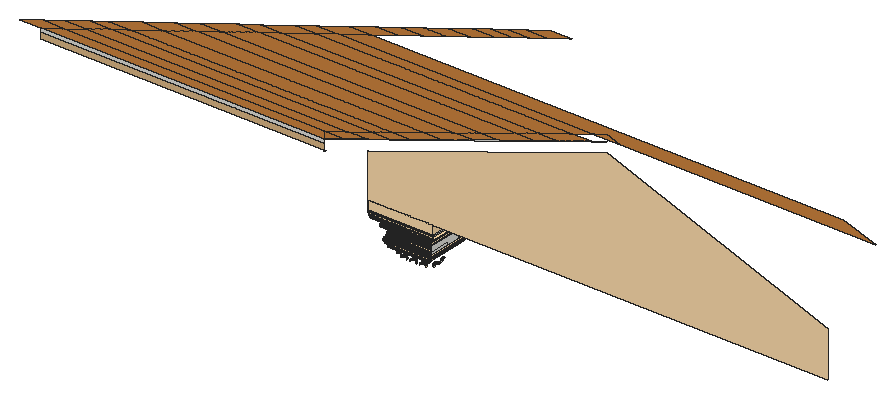
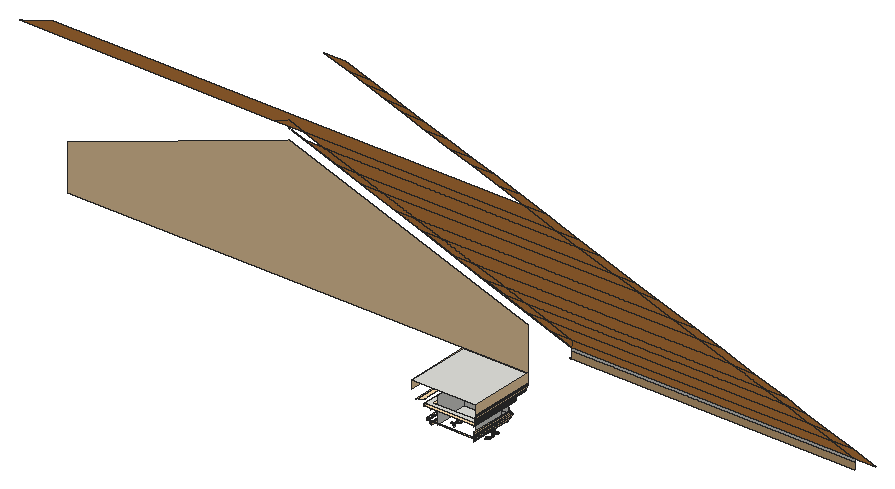
# SketchUp Ruby script. Lengths in inches.
U = 1.inch
M = Sketchup.active_model
def pt(a) = Geom::Point3d.new(a.map { |v| v * U })
def face(e, loops, mat)
  f = e.add_face(loops[0].map { |a| pt(a) })
  loops[1..].each { |l| e.add_face(l.map { |a| pt(a) }).erase! }
  f.material = f.back_material = mat if mat
  f
end
# faces: each face lists its corners as indices into pts; further lists are holes
def faces(e, pts, list, mat = nil) = list.each { |f| face(e, (f[0].is_a?(Array) ? f : [f]).map { |l| l.map { |i| pts[i] } }, mat) }
# xy, xz, yz: faces in a plane at the given z, y or x. An outline is a flat list of corners, or four numbers for a rectangle; further outlines are holes
def ring(l) = l.size == 4 ? [[l[0], l[1]], [l[2], l[1]], [l[2], l[3]], [l[0], l[3]]] : l.each_slice(2).to_a
def flat(e, list, mat, &to3) = list.each { |f| face(e, (f[0].is_a?(Array) ? f : [f]).map { |l| ring(l).map { |u, v| to3.(u, v) } }, mat) }
def xy(e, z, list, mat = nil) = flat(e, list, mat) { |x, y| [x, y, z] }
def xz(e, y, list, mat = nil) = flat(e, list, mat) { |x, z| [x, y, z] }
def yz(e, x, list, mat = nil) = flat(e, list, mat) { |y, z| [x, y, z] }
def lines(e, pts, list) = list.each { |a, b| e.add_line(pt(pts[a]), pt(pts[b])) }
# prism: a flat outline (further loops are holes) pulled along v
def prism(e, loops, v, mat = nil)
  f = face(e, loops, mat); d = Geom::Vector3d.new(v.map { |x| x * U })
  f.pushpull(f.normal.samedirection?(d) ? d.length : -d.length)
end
def box(e, o, s, mat = nil) = prism(e, [[o, [o[0] + s[0], o[1], o[2]], [o[0] + s[0], o[1] + s[1], o[2]], [o[0], o[1] + s[1], o[2]]]], [0, 0, s[2]], mat)
def at(x, y, z, deg = 0) = Geom::Transformation.translation(pt([x, y, z])) * Geom::Transformation.rotation(ORIGIN, Z_AXIS, deg.degrees)
def axes(o, x, y, z) = Geom::Transformation.new([*x, 0, *y, 0, *z, 0, *pt(o).to_a, 1])
def part(name) = M.definitions.add(name)
# library, detail: a bought-in or finely detailed component or shape, given as its bounding box
def library(name, o, s) = part(name).tap { |d| box(d.entities, o, s) }
def detail(e, o, s) = box(e.add_group.entities, o, s)
def put(e, d, t, mat = nil) = e.add_instance(d, t).tap { |i| i.material = mat if mat }
def group(e, t, mat = nil) = e.add_group.tap { |g| g.transformation = t; g.material = mat if mat }.entities
root = M.entities
M.materials.add("[0033_NavajoWhite]").color = [255, 222, 173]
M.materials.add("[0036_BurlyWood]").color = [222, 184, 135]
M.materials.add("[0040_Peru]").color = [205, 133, 63]
xy(root,95.99,[[110.21,8.1,123.2,14.59]])
xy(root,96.66,[[[109.62,7.51,123.79,21.68],[109.69,7.58,123.72,21.61]]],"[0033_NavajoWhite]")
xy(root,100.56,[[[109.03,6.92,124.38,22.27],[110.21,8.1,123.2,21.09]]],"[0033_NavajoWhite]")
xy(root,101.46,[[[109.03,6.92,124.38,22.27],[110.21,8.1,123.2,21.09]]])
xy(root,102.72,[[108.83,6.72,109.03,6.92,124.38,6.92,124.58,6.72]])
xy(root,102.72,[[108.04,5.93,108.04,23.25,108.83,22.47,109.03,22.27,109.03,6.92],[108.04,5.93,108.83,6.72,124.58,6.72,125.37,5.93],[125.37,5.93,124.38,6.92,124.38,22.27,124.58,22.47,125.37,23.25]],"[0033_NavajoWhite]")
xy(root,102.86,[[111,9.67,122.41,14.59]])
xy(root,105.42,[[108.83,6.72,124.58,14.59]])
xy(root,108.125,[[106.86,4.75,126.55,24.44]])
xz(root,4.75,[[93.16,116.81,93.71,117,93.16,117],[6.32,119,93.16,120],[93.16,119.98,93.21,120,93.16,120],[93.16,120,93.21,120,120.1,129.23,120.04,129.23,113.85,127.11,106.79,124.68,99.27,122.1],[120.04,129.23,120.1,129.23,139.33,135.83,139.26,135.83,129.4375,132.46],
  [139.26,135.83,139.33,135.83,147.21,138.54,147.13,138.54],[147.13,138.54,147.21,138.54,164.92,144.62,164.84,144.62,157.86,142.22],[164.84,144.62,164.92,144.62,180,149.8,179.96,149.82,175.27,148.21]])
xz(root,4.75,[[106.86,105.42,126.55,108.125],[106.86,108.125,247.8,108.125,247.8,122.125,179.96,146.625,106.86,121.52]],"[0033_NavajoWhite]")
xz(root,4.75,[[6.32,117,93.16,119]],"[0036_BurlyWood]")
xz(root,4.75,[[0,120,6.32,120,13.35,122.34,7.02,122.34],[6.32,120,93.16,120,93.16,122.1,13.35,122.34],[93.16,120,99.27,122.1,93.16,122.1],[93.16,122.1,100.6875,124.68,20.37,124.68,13.35,122.34],[93.16,122.1,99.27,122.1,106.79,124.68,100.6875,124.68],
  [7.02,122.34,13.35,122.34,20.37,124.68,14.04,124.68],[14.04,124.68,20.37,124.68,27.65,127.11,21.32,127.11],[20.37,124.68,100.6875,124.68,107.75,127.11,27.65,127.11],[100.6875,124.68,106.79,124.68,113.85,127.11,107.75,127.11],[21.32,127.11,27.65,127.11,33.71,129.13,27.39,129.13],
  [27.65,127.11,107.75,127.11,113.9375,129.23,33.71,129.13],[107.75,127.11,113.85,127.11,120.04,129.23,113.9375,129.23],[27.39,129.13,33.71,129.13,43.71,132.46,37.38,132.46],[33.71,129.13,113.9375,129.23,123.33,132.46,43.71,132.46],[113.9375,129.23,120.04,129.23,129.4375,132.46,123.33,132.46],
  [37.38,132.46,43.71,132.46,53.83,135.83,47.5,135.83],[43.71,132.46,123.33,132.46,133.15,135.83,53.83,135.83],[123.33,132.46,129.4375,132.46,139.26,135.83,133.15,135.83],[47.5,135.83,53.83,135.83,61.94,138.54,55.62,138.54],[53.83,135.83,133.15,135.83,141.03,138.54,61.94,138.54],
  [133.15,135.83,139.26,135.83,147.13,138.54,141.03,138.54],[55.62,138.54,61.94,138.54,73,142.22,66.67,142.22],[61.94,138.54,141.03,138.54,151.75,142.22,73,142.22],[141.03,138.54,147.13,138.54,157.86,142.22,151.75,142.22],[66.67,142.22,73,142.22,80.19,144.62,73.87,144.62],
  [73,142.22,151.75,142.22,158.73,144.62,80.19,144.62],[151.75,142.22,157.86,142.22,164.84,144.62,158.73,144.62],[73.87,144.62,80.19,144.62,90.94,148.21,84.62,148.21],[80.19,144.62,158.73,144.62,169.17,148.21,90.94,148.21],[158.73,144.62,164.84,144.62,175.27,148.21,169.17,148.21],
  [84.62,148.21,90.94,148.21,97.46,150.38,91.14,150.38],[90.94,148.21,169.17,148.21,175.49,150.38,97.46,150.38],[91.14,150.38,97.46,150.38,107.66,153.78,101.33,153.78],[97.46,150.38,175.49,150.38,180,151.93,184.29,150.38,262.54,150.38,252.34,153.78,107.66,153.78],[175.49,150.38,184.29,150.38,180,151.93],
  [101.33,153.78,107.66,153.78,115.67,156.45,109.34,156.45],[109.34,156.45,115.67,156.45,123.61,159.09,117.28,159.09],[117.28,159.09,123.61,159.09,130.36,161.35,124.04,161.35],[124.04,161.35,130.36,161.35,137.99,163.89,131.67,163.89],[131.67,163.89,137.99,163.89,145.25,166.31,138.93,166.31],
  [138.93,166.31,145.25,166.31,150.49,168.05,144.16,168.05],[144.16,168.05,150.49,168.05,156.26,169.98,149.93,169.98],[149.93,169.98,156.26,169.98,161.41,171.69,155.08,171.69],[155.08,171.69,161.41,171.69,169.18,174.29,162.86,174.29]],"[0040_Peru]")
xz(root,6.72,[[108.83,102.72,124.58,105.42]])
xz(root,7.11,[[109.22,101.95,124.19,101.95,124.1875,102.09,109.23,102.09],[109.23,102.09,124.1875,102.09,124.19,102.23,109.22,102.23]],"[0033_NavajoWhite]")
xz(root,7.58,[[109.69,95.99,123.72,96.66]],"[0033_NavajoWhite]")
xz(root,8.1,[[110.21,94.95,123.2,95.1],[110.21,95.1,123.2,95.99],[110.21,95.99,123.2,97.5625],[110.21,97.5625,123.2,99.87],[110.21,99.87,123.2,100.56],
  [110.21,100.56,123.2,101.46]])
xz(root,9.67,[[111,94.95,122.41,102.86]])
yz(root,106.86,[[4.75,105.42,24.44,108.125]],"[0033_NavajoWhite]")
yz(root,110.21,[[8.1,95.99,14.59,97.5625]])
yz(root,111,[[9.67,94.95,19.51,102.86]])
yz(root,122.41,[[9.67,94.95,19.51,102.86]])
yz(root,123.2,[[8.1,95.99,14.59,97.5625]])
yz(root,126.55,[[4.75,105.42,24.44,108.125]],"[0033_NavajoWhite]")
p = [[112.83,9.92,92.48],[112.8,9.67,92.48],[112.77,9.67,92.25],[112.8,9.93,92.25],[114.7,9.93,92.25],[114.74,9.67,92.25],
  [114.7,9.67,92.48],[114.67,9.92,92.48],[115.79,9.92,92.48],[115.76,9.67,92.48],[115.72,9.67,92.25],[115.76,9.93,92.25],
  [117.66,9.93,92.25],[117.69,9.67,92.25],[117.66,9.67,92.48],[117.625,9.92,92.48],[118.74,9.92,92.48],[118.71,9.67,92.48],
  [118.67,9.67,92.25],[118.71,9.93,92.25],[120.61,9.93,92.25],[120.64,9.67,92.25],[120.61,9.67,92.48],[120.58,9.92,92.48],
  [112.9,10.16,92.25],[112.93,10.15,92.48],[114.58,10.15,92.48],[114.61,10.16,92.25],[115.85,10.16,92.25],[115.88,10.15,92.48],
  [117.53,10.15,92.48],[117.56,10.16,92.25],[118.81,10.16,92.25],[118.84,10.15,92.48],[120.48,10.15,92.48],[120.51,10.16,92.25],
  [113.06,10.37,92.25],[113.08,10.34,92.48],[114.43,10.34,92.48],[114.45,10.37,92.25],[116.01,10.37,92.25],[116.03,10.34,92.48],
  [117.38,10.34,92.48],[117.4,10.37,92.25],[118.96,10.37,92.25],[118.99,10.34,92.48],[120.33,10.34,92.48],[120.35,10.37,92.25],
  [113.26,10.52,92.25],[113.28,10.49,92.48],[114.23,10.49,92.48],[114.25,10.52,92.25],[116.21,10.52,92.25],[116.23,10.49,92.48],
  [117.18,10.49,92.48],[117.2,10.52,92.25],[119.17,10.52,92.25],[119.18,10.49,92.48],[120.13,10.49,92.48],[120.15,10.52,92.25],
  [113.5,10.62,92.25],[113.51,10.59,92.48],[114,10.59,92.48],[114.01,10.62,92.25],[116.45,10.62,92.25],[116.46,10.59,92.48],
  [116.95,10.59,92.48],[116.96,10.62,92.25],[119.4,10.62,92.25],[119.41,10.59,92.48],[119.9,10.59,92.48],[119.91,10.62,92.25],
  [113.75,10.66,92.25],[113.75,10.62,92.48],[116.71,10.66,92.25],[116.71,10.62,92.48],[119.66,10.66,92.25],[119.66,10.62,92.48],
  [112.93,9.89,92.7],[112.9,9.67,92.7],[114.61,9.67,92.7],[114.58,9.89,92.7],[115.88,9.89,92.7],[115.85,9.67,92.7],
  [117.56,9.67,92.7],[117.53,9.89,92.7],[118.84,9.89,92.7],[118.81,9.67,92.7],[120.51,9.67,92.7],[120.48,9.89,92.7],
  [113.01,10.1,92.7],[114.49,10.1,92.7],[115.97,10.1,92.7],[117.44,10.1,92.7],[118.92,10.1,92.7],[120.4,10.1,92.7],
  [113.15,10.27,92.7],[114.36,10.27,92.7],[116.1,10.27,92.7],[117.31,10.27,92.7],[119.06,10.27,92.7],[120.26,10.27,92.7],
  [113.33,10.41,92.7],[114.18,10.41,92.7],[116.28,10.41,92.7],[117.13,10.41,92.7],[119.23,10.41,92.7],[120.08,10.41,92.7],
  [113.53,10.49,92.7],[113.97,10.49,92.7],[116.49,10.49,92.7],[116.93,10.49,92.7],[119.4375,10.49,92.7],[119.88,10.49,92.7],
  [113.75,10.52,92.7],[116.71,10.52,92.7],[119.66,10.52,92.7],[111.25,10.6875,92.51],[111,10.66,92.51],[111,10.6875,92.74],
  [111.24,10.72,92.74],[111.47,10.82,92.74],[111.49,10.79,92.51],[121.92,10.79,92.51],[121.9375,10.82,92.74],[122.17,10.72,92.74],
  [122.16,10.6875,92.51],[122.41,10.66,92.51],[122.41,10.6875,92.74],[111.67,10.97,92.74],[111.69,10.94,92.51],[121.72,10.94,92.51],
  [121.74,10.97,92.74],[111.82,11.16,92.74],[111.85,11.15,92.51],[121.5625,11.15,92.51],[121.59,11.16,92.74],[111.92,11.39,92.74],
  [111.95,11.39,92.51],[121.46,11.39,92.51],[121.5,11.39,92.74],[111.95,11.64,92.74],[111.98,11.64,92.51],[121.43,11.64,92.51],
  [121.46,11.64,92.74],[111.92,11.89,92.74],[111.95,11.89,92.51],[121.46,11.89,92.51],[121.5,11.89,92.74],[111.82,12.12,92.74],
  [111.85,12.13,92.51],[121.5625,12.13,92.51],[121.59,12.12,92.74],[111.67,12.3125,92.74],[111.69,12.34,92.51],[121.72,12.34,92.51],
  [121.74,12.3125,92.74],[111.47,12.46,92.74],[111.49,12.49,92.51],[121.92,12.49,92.51],[121.9375,12.46,92.74],[111.24,12.56,92.74],
  [111.25,12.59,92.51],[122.16,12.59,92.51],[122.17,12.56,92.74],[111,12.59,92.74],[111,12.625,92.51],[122.41,12.59,92.74],
  [122.41,12.625,92.51],[111.25,13.64,92.51],[111,13.61,92.51],[111,13.64,92.74],[111.24,13.67,92.74],[111.47,13.77,92.74],
  [111.49,13.74,92.51],[121.92,13.74,92.51],[121.9375,13.77,92.74],[122.17,13.67,92.74],[122.16,13.64,92.51],[122.41,13.61,92.51],
  [122.41,13.64,92.74],[111.67,13.92,92.74],[111.69,13.9,92.51],[121.72,13.9,92.51],[121.74,13.92,92.74],[111.82,14.12,92.74],
  [111.85,14.1,92.51],[121.5625,14.1,92.51],[121.59,14.12,92.74],[111.92,14.35,92.74],[111.95,14.34,92.51],[121.46,14.34,92.51],
  [121.5,14.35,92.74],[111.95,14.59,92.74],[111.98,14.59,92.51],[121.43,14.59,92.51],[121.46,14.59,92.74],[113.08,9.85,92.89],
  [113.06,9.67,92.89],[114.45,9.67,92.89],[114.43,9.85,92.89],[116.03,9.85,92.89],[116.01,9.67,92.89],[117.4,9.67,92.89],
  [117.38,9.85,92.89],[118.99,9.85,92.89],[118.96,9.67,92.89],[120.35,9.67,92.89],[120.33,9.85,92.89],[113.15,10.02,92.89],
  [114.36,10.02,92.89],[116.1,10.02,92.89],[117.31,10.02,92.89],[119.06,10.02,92.89],[120.26,10.02,92.89],[113.26,10.16,92.89],
  [114.25,10.16,92.89],[116.21,10.16,92.89],[117.2,10.16,92.89],[119.17,10.16,92.89],[120.15,10.16,92.89],[113.41,10.27,92.89],
  [114.1,10.27,92.89],[116.36,10.27,92.89],[117.05,10.27,92.89],[119.3125,10.27,92.89],[120.01,10.27,92.89],[113.57,10.34,92.89],
  [113.75,10.37,92.89],[113.93,10.34,92.89],[116.53,10.34,92.89],[116.71,10.37,92.89],[116.89,10.34,92.89],[119.48,10.34,92.89],
  [119.66,10.37,92.89],[119.84,10.34,92.89],[111,10.79,92.96],[111.22,10.82,92.96],[111.42,10.9,92.96],[121.99,10.9,92.96],
  [122.19,10.82,92.96],[122.41,10.79,92.96],[111.6,11.04,92.96],[121.8125,11.04,92.96],[111.74,11.21,92.96],[121.68,11.21,92.96],
  [111.82,11.42,92.96],[121.59,11.42,92.96],[111.85,11.64,92.96],[121.5625,11.64,92.96],[111.82,11.86,92.96],[121.59,11.86,92.96],
  [111.74,12.07,92.96],[121.68,12.07,92.96],[111.6,12.24,92.96],[121.8125,12.24,92.96],[111.42,12.38,92.96],[121.99,12.38,92.96],
  [111.22,12.46,92.96],[122.19,12.46,92.96],[111,12.49,92.96],[122.41,12.49,92.96],[111,13.74,92.96],[111.22,13.77,92.96],
  [122.19,13.77,92.96],[122.41,13.74,92.96],[111.42,13.85,92.96],[121.99,13.85,92.96],[111.6,13.99,92.96],[121.8125,13.99,92.96],
  [111.74,14.17,92.96],[121.68,14.17,92.96],[111.82,14.37,92.96],[121.59,14.37,92.96],[111.85,14.59,92.96],[121.5625,14.59,92.96],
  [113.28,9.8,93.03],[113.26,9.67,93.03],[114.25,9.67,93.03],[114.23,9.8,93.03],[116.23,9.8,93.03],[116.21,9.67,93.03],
  [117.2,9.67,93.03],[117.18,9.8,93.03],[119.18,9.8,93.03],[119.17,9.67,93.03],[120.15,9.67,93.03],[120.13,9.8,93.03],
  [113.33,9.92,93.03],[114.18,9.92,93.03],[116.28,9.92,93.03],[117.13,9.92,93.03],[119.23,9.92,93.03],[120.08,9.92,93.03],
  [113.41,10.02,93.03],[114.1,10.02,93.03],[116.36,10.02,93.03],[117.05,10.02,93.03],[119.3125,10.02,93.03],[120.01,10.02,93.03],
  [113.51,10.1,93.03],[114,10.1,93.03],[116.46,10.1,93.03],[116.95,10.1,93.03],[119.41,10.1,93.03],[119.9,10.1,93.03],
  [113.625,10.15,93.03],[113.75,10.16,93.03],[113.88,10.15,93.03],[116.58,10.15,93.03],[116.71,10.16,93.03],[116.83,10.15,93.03],
  [119.53,10.15,93.03],[119.66,10.16,93.03],[119.79,10.15,93.03],[113.51,9.74,93.12],[113.5,9.67,93.12],[113.53,9.8,93.12],
  [114.01,9.67,93.12],[114,9.74,93.12],[113.97,9.8,93.12],[116.46,9.74,93.12],[116.45,9.67,93.12],[116.49,9.8,93.12],
  [116.93,9.8,93.12],[116.95,9.74,93.12],[116.96,9.67,93.12],[119.41,9.74,93.12],[119.4,9.67,93.12],[119.4375,9.8,93.12],
  [119.91,9.67,93.12],[119.9,9.74,93.12],[119.88,9.8,93.12],[113.57,9.85,93.12],[113.93,9.85,93.12],[116.53,9.85,93.12],
  [116.89,9.85,93.12],[119.48,9.85,93.12],[119.84,9.85,93.12],[113.625,9.89,93.12],[113.6875,9.92,93.12],[113.75,9.93,93.12],
  [113.82,9.92,93.12],[113.88,9.89,93.12],[116.58,9.89,93.12],[116.64,9.92,93.12],[116.71,9.93,93.12],[116.77,9.92,93.12],
  [116.83,9.89,93.12],[119.53,9.89,93.12],[119.59,9.92,93.12],[119.66,9.93,93.12],[119.72,9.92,93.12],[119.79,9.89,93.12],
  [111,10.94,93.15],[111.18,10.97,93.15],[111.35,11.04,93.15],[122.07,11.04,93.15],[122.23,10.97,93.15],[122.41,10.94,93.15],
  [111.49,11.15,93.15],[121.92,11.15,93.15],[111.6,11.29,93.15],[121.8125,11.29,93.15],[111.67,11.46,93.15],[121.74,11.46,93.15],
  [111.69,11.64,93.15],[121.72,11.64,93.15],[111.67,11.82,93.15],[121.74,11.82,93.15],[111.6,11.99,93.15],[121.8125,11.99,93.15],
  [111.49,12.13,93.15],[121.92,12.13,93.15],[111.35,12.24,93.15],[122.07,12.24,93.15],[111.18,12.3125,93.15],[122.23,12.3125,93.15],
  [111,12.34,93.15],[122.41,12.34,93.15],[111,13.9,93.15],[111.18,13.92,93.15],[122.23,13.92,93.15],[122.41,13.9,93.15],
  [111.35,13.99,93.15],[122.07,13.99,93.15],[111.49,14.1,93.15],[121.92,14.1,93.15],[111.6,14.24,93.15],[121.8125,14.24,93.15],
  [111.67,14.41,93.15],[121.74,14.41,93.15],[111.69,14.59,93.15],[121.72,14.59,93.15],[113.75,9.67,93.15],[116.71,9.67,93.15],
  [119.66,9.67,93.15],[111,11.15,93.29],[111.125,11.16,93.29],[122.29,11.16,93.29],[122.41,11.15,93.29],[111.24,11.21,93.29],
  [111.35,11.29,93.29],[122.07,11.29,93.29],[122.17,11.21,93.29],[111.42,11.39,93.29],[121.99,11.39,93.29],[111.47,11.51,93.29],
  [121.9375,11.51,93.29],[111.49,11.64,93.29],[121.92,11.64,93.29],[111.47,11.77,93.29],[121.9375,11.77,93.29],[111.42,11.89,93.29],
  [121.99,11.89,93.29],[111.35,11.99,93.29],[122.07,11.99,93.29],[111.24,12.07,93.29],[122.17,12.07,93.29],[111.125,12.12,93.29],
  [111,12.13,93.29],[122.29,12.12,93.29],[122.41,12.13,93.29],[111,14.1,93.29],[111.125,14.12,93.29],[111.24,14.17,93.29],
  [122.17,14.17,93.29],[122.29,14.12,93.29],[122.41,14.1,93.29],[111.35,14.24,93.29],[122.07,14.24,93.29],[111.42,14.35,93.29],
  [121.99,14.35,93.29],[111.47,14.47,93.29],[121.9375,14.47,93.29],[111.49,14.59,93.29],[121.92,14.59,93.29],[111,11.39,93.38],
  [111.0625,11.39,93.38],[122.35,11.39,93.38],[122.41,11.39,93.38],[111.125,11.42,93.38],[111.18,11.46,93.38],[122.23,11.46,93.38],
  [122.29,11.42,93.38],[111.22,11.51,93.38],[122.19,11.51,93.38],[111.24,11.57,93.38],[122.17,11.57,93.38],[111.25,11.64,93.38],
  [122.16,11.64,93.38],[111.24,11.71,93.38],[122.17,11.71,93.38],[111.22,11.77,93.38],[122.19,11.77,93.38],[111.125,11.86,93.38],
  [111.18,11.82,93.38],[122.23,11.82,93.38],[122.29,11.86,93.38],[111.0625,11.89,93.38],[111,11.89,93.38],[122.35,11.89,93.38],
  [122.41,11.89,93.38],[111,14.34,93.38],[111.0625,14.35,93.38],[111.125,14.37,93.38],[122.29,14.37,93.38],[122.35,14.35,93.38],
  [122.41,14.34,93.38],[111.18,14.41,93.38],[111.22,14.47,93.38],[122.19,14.47,93.38],[122.23,14.41,93.38],[111.24,14.53,93.38],
  [122.17,14.53,93.38],[111.25,14.59,93.38],[122.16,14.59,93.38],[111,11.64,93.41],[122.41,11.64,93.41],[111,14.59,93.41],
  [122.41,14.59,93.41],[110.2,8.09,95.25],[110.21,8.1,95.1],[123.2,8.1,95.1],[123.21,8.09,95.25],[110.18,8.06,95.4],
  [123.23,8.06,95.4],[110.15,8.03,95.53],[123.26,8.03,95.53],[110.15,21.15,95.53],[110.18,21.12,95.4],[123.23,21.12,95.4],
  [123.26,21.15,95.53],[110.11,8,95.66],[123.3,8,95.66],[110.11,21.1875,95.66],[123.3,21.1875,95.66],[110.0625,7.95,95.77],
  [123.35,7.95,95.77],[110.0625,21.24,95.77],[123.35,21.24,95.77],[110.01,7.9,95.86],[123.4,7.9,95.86],[109.89,7.78,95.98],
  [109.95,7.84,95.93],[123.46,7.84,95.93],[123.52,7.78,95.98],[109.89,21.41,95.98],[109.95,21.35,95.93],[123.46,21.35,95.93],
  [123.52,21.41,95.98],[109.86,7.74,95.99],[123.55,7.74,95.99],[109.48,7.37,96.79],[109.52,7.41,96.72],[123.89,7.41,96.72],
  [123.93,7.37,96.79],[109.57,7.45,96.68],[123.84,7.45,96.68],[109.48,21.82,96.79],[109.52,21.78,96.72],[109.57,21.73,96.68],
  [123.89,21.78,96.72],[123.93,21.82,96.79],[109.62,7.51,96.66],[123.79,7.51,96.66],[109.62,21.68,96.66],[109.45,7.34,96.89],
  [123.96,7.34,96.89],[109.45,21.85,96.89],[123.96,21.85,96.89],[109.43,7.32,96.99],[123.98,7.32,96.99],[109.43,21.87,96.99],
  [109.42,7.31,97.11],[123.99,7.31,97.11],[109.42,21.875,97.11],[109.43,7.32,97.23],[123.98,7.32,97.23],[109.43,21.87,97.23],
  [109.45,7.34,97.34],[123.96,7.34,97.34],[109.45,21.85,97.34],[109.48,7.37,97.43],[123.93,7.37,97.43],[109.48,21.82,97.43],
  [123.96,21.85,97.34],[123.93,21.82,97.43],[109.52,7.41,97.5],[123.89,7.41,97.5],[109.52,21.78,97.5],[123.89,21.78,97.5],
  [109.57,7.45,97.55],[123.84,7.45,97.55],[109.57,21.73,97.55],[109.62,7.51,97.5625],[123.79,7.51,97.5625],[109.62,21.68,97.5625],
  [109.72,7.61,97.74],[123.69,7.61,97.74],[109.72,21.58,97.74],[109.8125,7.7,97.93],[123.6,7.7,97.93],[109.9,7.78,98.14],
  [123.52,7.78,98.14],[109.9,21.4,98.14],[109.8125,21.49,97.93],[109.97,7.86,98.375],[123.44,7.86,98.375],[110.04,7.92,98.62],
  [123.375,7.92,98.62],[110.09,7.98,98.875],[123.32,7.98,98.875],[110.14,8.03,99.14],[123.27,8.03,99.14],[110.18,8.0625,99.42],
  [123.24,8.0625,99.42],[110.2,8.09,99.7],[123.21,8.09,99.7],[110.2,21.1,99.7],[110.18,21.12,99.42],[123.24,21.12,99.42],
  [123.21,21.1,99.7],[110.21,8.1,99.87],[123.2,8.1,99.87],[108.89,6.78,100.6875],[108.93,6.82,100.62],[124.48,6.82,100.62],
  [124.52,6.78,100.6875],[108.98,6.86,100.57],[124.43,6.86,100.57],[109.03,6.92,100.56],[124.38,6.92,100.56],[108.98,22.32,100.57],
  [109.03,22.27,100.56],[108.86,6.74,100.78],[124.55,6.74,100.78],[108.86,22.44,100.78],[108.89,22.41,100.6875],[108.84,6.73,100.89],
  [124.57,6.73,100.89],[108.84,22.46,100.89],[124.55,22.44,100.78],[124.57,22.46,100.89],[108.83,6.72,101.01],[124.58,6.72,101.01],
  [108.83,22.47,101.01],[108.84,6.73,101.125],[124.57,6.73,101.125],[108.84,22.46,101.125],[108.86,6.74,101.23],[124.55,6.74,101.23],
  [108.86,22.44,101.23],[124.57,22.46,101.125],[124.55,22.44,101.23],[108.89,6.78,101.33],[124.52,6.78,101.33],[108.89,22.41,101.33],
  [108.93,6.82,101.4],[124.48,6.82,101.4],[108.98,6.86,101.44],[124.43,6.86,101.44],[109.03,6.92,101.46],[124.38,6.92,101.46],
  [109.03,22.27,101.46],[108.98,22.32,101.44],[124.33,6.97,101.52],[109.08,6.97,101.52],[109.08,22.22,101.52],[124.33,22.22,101.52],
  [124.38,22.27,101.46],[124.28,7.02,101.6],[109.13,7.02,101.6],[109.13,22.17,101.6],[124.24,7.06,101.7],[109.17,7.06,101.7],
  [109.17,22.13,101.7],[124.21,7.09,101.82],[109.2,7.09,101.82],[109.2,22.1,101.82],[124.19,7.11,101.95],[109.22,7.11,101.95],
  [124.19,7.11,102.23],[124.21,7.09,102.36],[109.2,7.09,102.36],[109.22,7.11,102.23],[124.24,7.06,102.48],[109.17,7.06,102.48],
  [109.2,22.1,102.36],[109.17,22.13,102.48],[124.28,7.02,102.58],[109.13,7.02,102.58],[109.13,22.17,102.58],[124.33,6.97,102.66],
  [109.08,6.97,102.66],[109.08,22.22,102.66],[125.6875,5.61,102.73],[125.85,5.45,102.82],[107.57,5.45,102.82],[107.72,5.61,102.73],
  [107.57,23.73,102.82],[107.72,23.58,102.73],[125.6875,23.58,102.73],[125.85,23.73,102.82],[125.53,5.77,102.7],[107.88,5.77,102.7],
  [107.88,23.41,102.7],[125.37,5.93,102.72],[108.04,5.93,102.72],[108.04,23.25,102.72],[124.38,6.92,102.72],[109.03,6.92,102.72],
  [109.03,22.27,102.72],[124.38,22.27,102.72],[124.33,22.22,102.66],[125.99,5.3,102.96],[107.42,5.3,102.96],[107.42,23.88,102.96],
  [126.13,5.17,103.15],[107.28,5.17,103.15],[126.25,5.05,103.39],[107.16,5.05,103.39],[107.16,24.14,103.39],[107.28,24.02,103.15],
  [126.36,4.94,103.68],[107.05,4.94,103.68],[107.05,24.24,103.68],[126.44,4.86,103.99],[106.97,4.86,103.99],[126.51,4.79,104.33],
  [106.91,4.79,104.33],[106.91,24.39,104.33],[106.97,24.33,103.99],[126.54,4.75,104.6875],[106.87,4.75,104.6875],[106.87,24.43,104.6875],
  [126.56,4.74,105.05],[106.85,4.74,105.05],[126.55,4.75,105.42],[106.86,4.75,105.42],[106.86,24.44,105.42],[106.85,24.45,105.05]]
faces(root,p,[[0,1,2,3],[4,5,6,7],[8,9,10,11],[12,13,14,15],[16,17,18,19],[20,21,22,23],[0,3,24,25],[26,27,4,7],
  [8,11,28,29],[30,31,12,15],[16,19,32,33],[34,35,20,23],[25,24,36,37],[38,39,27,26],[29,28,40,41],[42,43,31,30],
  [33,32,44,45],[46,47,35,34],[37,36,48,49],[50,51,39,38],[41,40,52,53],[54,55,43,42],[45,44,56,57],[58,59,47,46],
  [49,48,60,61],[62,63,51,50],[53,52,64,65],[66,67,55,54],[57,56,68,69],[70,71,59,58],[61,60,72,73],[73,72,63,62],
  [65,64,74,75],[75,74,67,66],[69,68,76,77],[77,76,71,70],[78,79,1,0],[7,6,80,81],[82,83,9,8],[15,14,84,85],
  [86,87,17,16],[23,22,88,89],[78,0,25,90],[91,26,7,81],[82,8,29,92],[93,30,15,85],[86,16,33,94],[95,34,23,89],
  [90,25,37,96],[97,38,26,91],[92,29,41,98],[99,42,30,93],[94,33,45,100],[101,46,34,95],[96,37,49,102],[103,50,38,97],
  [98,41,53,104],[105,54,42,99],[100,45,57,106],[107,58,46,101],[102,49,61,108],[109,62,50,103],[104,53,65,110],[111,66,54,105],
  [106,57,69,112],[113,70,58,107],[108,61,73,114],[114,73,62,109],[110,65,75,115],[115,75,66,111],[112,69,77,116],[116,77,70,113],
  [197,198,79,78],[81,80,199,200],[201,202,83,82],[85,84,203,204],[205,206,87,86],[89,88,207,208],[197,78,90,209],[210,91,81,200],
  [201,82,92,211],[212,93,85,204],[205,86,94,213],[214,95,89,208],[209,90,96,215],[216,97,91,210],[211,92,98,217],[218,99,93,212],
  [213,94,100,219],[220,101,95,214],[215,96,102,221],[222,103,97,216],[217,98,104,223],[224,105,99,218],[219,100,106,225],[226,107,101,220],
  [221,102,108,227],[227,108,114,228],[228,114,109,229],[229,109,103,222],[223,104,110,230],[230,110,115,231],[231,115,111,232],[232,111,105,224],
  [225,106,112,233],[233,112,116,234],[234,116,113,235],[235,113,107,226],[276,277,198,197],[200,199,278,279],[280,281,202,201],[204,203,282,283],
  [284,285,206,205],[208,207,286,287],[276,197,209,288],[289,210,200,279],[280,201,211,290],[291,212,204,283],[284,205,213,292],[293,214,208,287],
  [288,209,215,294],[295,216,210,289],[290,211,217,296],[297,218,212,291],[292,213,219,298],[299,220,214,293],[294,215,221,300],[301,222,216,295],
  [296,217,223,302],[303,224,218,297],[298,219,225,304],[305,226,220,299],[300,221,227,306],[306,227,228,307],[307,228,229,308],[308,229,222,301],
  [302,223,230,309],[309,230,231,310],[310,231,232,311],[311,232,224,303],[304,225,233,312],[312,233,234,313],[313,234,235,314],[314,235,226,305],
  [315,316,277,276],[315,276,288,317],[279,278,318,319],[320,289,279,319],[321,322,281,280],[321,280,290,323],[324,291,283,325],[283,282,326,325],
  [327,328,285,284],[327,284,292,329],[287,286,330,331],[332,293,287,331],[317,288,294,333],[334,295,289,320],[323,290,296,335],[336,297,291,324],
  [329,292,298,337],[338,299,293,332],[333,294,300,339],[339,300,306,340],[340,306,307,341],[342,308,301,343],[341,307,308,342],[343,301,295,334],
  [335,296,302,344],[344,302,309,345],[345,309,310,346],[346,310,311,347],[348,303,297,336],[347,311,303,348],[337,298,304,349],[349,304,312,350],
  [350,312,313,351],[352,314,305,353],[351,313,314,352],[353,305,299,338],[315,394,316],[394,315,317],[394,317,333],[394,333,339],
  [394,339,340],[394,340,341],[319,318,394],[394,320,319],[394,334,320],[394,343,334],[394,342,343],[394,341,342],
  [321,395,322],[395,321,323],[395,323,335],[395,335,344],[395,344,345],[395,345,346],[325,326,395],[395,324,325],
  [395,336,324],[395,348,336],[395,347,348],[395,346,347],[327,396,328],[396,327,329],[396,329,337],[396,337,349],
  [396,349,350],[396,350,351],[331,330,396],[396,332,331],[396,338,332],[396,353,338],[396,352,353],[396,351,352],
  [481,482,483,484],[485,481,484,486],[487,485,486,488],[487,489,490,485],[486,491,492,488],[493,487,488,494],[493,495,489,487],[488,492,496,494],
  [497,493,494,498],[497,499,495,493],[494,496,500,498],[501,497,498,502],[503,504,505,506],[503,507,508,504],[504,501,502,505],[505,509,510,506],
  [511,503,506,512],[513,514,515,516],[514,517,518,515],[513,519,520,514],[514,520,521,517],[515,522,523,516],[517,524,525,518],[517,521,526,524],
  [527,513,516,528],[527,529,519,513],[516,523,530,528],[531,527,528,532],[531,533,529,527],[534,531,532,535],[534,536,533,531],[537,534,535,538],
  [537,539,536,534],[540,537,538,541],[540,542,539,537],[543,540,541,544],[543,545,542,540],[541,546,547,544],[548,543,544,549],[548,550,545,543],
  [544,547,551,549],[552,548,549,553],[552,554,550,548],[555,552,553,556],[555,557,554,552],[558,555,556,559],[558,560,557,555],[561,558,559,562],
  [563,561,562,564],[563,565,566,561],[567,563,564,568],[569,567,568,570],[571,569,570,572],[573,571,572,574],[575,573,574,576],[577,575,576,578],
  [579,580,575,577],[576,581,582,578],[583,577,578,584],[585,586,587,588],[586,589,590,587],[589,591,592,590],[589,593,594,591],[595,585,588,596],
  [595,597,598,585],[599,595,596,600],[599,601,597,595],[596,602,603,600],[604,599,600,605],[604,606,601,599],[607,604,605,608],[607,609,606,604],
  [610,607,608,611],[610,612,609,607],[613,614,611,608],[615,610,611,616],[615,617,612,610],[618,615,616,619],[620,618,619,621],[622,620,621,623],
  [622,624,625,620],[623,626,627,622],[626,631,632,627],[631,634,635,632],[634,637,638,635],[637,640,641,638],[642,643,644,645],[643,646,647,644],
  [646,650,651,647],[650,653,654,651],[656,657,658,659],[658,660,661,659],[656,662,663,657],[664,656,659,665],[659,661,666,665],[667,664,665,668],
  [665,666,669,668],[653,670,671,654],[657,675,676,658],[676,677,660,658],[675,678,679,676],[678,680,681,679],[681,682,683,679],[680,684,685,681],
  [685,686,682,681],[684,687,688,685],[687,689,690,688],[690,691,692,688],[689,693,694,690],[694,695,691,690],[693,696,697,694],[696,698,699,697],
  [699,700,701,697]],"[0033_NavajoWhite]")
faces(root,p,[[117,118,119,120],[121,122,117,120],[123,124,125,126],[127,126,125,128],[129,130,122,121],[131,132,124,123],[133,134,130,129],[135,136,132,131],
  [137,138,134,133],[139,140,136,135],[141,142,138,137],[143,144,140,139],[145,146,142,141],[147,148,144,143],[149,150,146,145],[151,152,148,147],
  [153,154,150,149],[155,156,152,151],[157,158,154,153],[159,160,156,155],[161,162,158,157],[163,164,160,159],[161,165,166,162],[167,164,163,168],
  [169,170,171,172],[173,174,169,172],[175,176,177,178],[179,178,177,180],[181,182,174,173],[183,184,176,175],[185,186,182,181],[187,188,184,183],
  [189,190,186,185],[191,192,188,187],[193,194,190,189],[195,196,192,191],[120,119,236,237],[238,121,120,237],[124,239,240,125],[128,125,240,241],
  [242,129,121,238],[132,243,239,124],[244,133,129,242],[136,245,243,132],[246,137,133,244],[140,247,245,136],[248,141,137,246],[144,249,247,140],
  [250,145,141,248],[148,251,249,144],[252,149,145,250],[152,253,251,148],[254,153,149,252],[156,255,253,152],[256,157,153,254],[160,257,255,156],
  [258,161,157,256],[164,259,257,160],[258,260,165,161],[261,259,164,167],[172,171,262,263],[180,177,264,265],[266,173,172,263],[176,267,264,177],
  [268,181,173,266],[184,269,267,176],[270,185,181,268],[188,271,269,184],[272,189,185,270],[192,273,271,188],[274,193,189,272],[196,275,273,192],
  [237,236,354,355],[356,238,237,355],[239,357,358,240],[241,240,358,359],[360,242,238,356],[243,361,357,239],[362,244,242,360],[245,363,361,243],
  [364,246,244,362],[247,365,363,245],[366,248,246,364],[249,367,365,247],[368,250,248,366],[251,369,367,249],[370,252,250,368],[253,371,369,251],
  [372,254,252,370],[255,373,371,253],[374,256,254,372],[257,375,373,255],[376,258,256,374],[259,377,375,257],[376,378,260,258],[379,377,259,261],
  [263,262,380,381],[265,264,382,383],[384,266,263,381],[267,385,382,264],[386,268,266,384],[269,387,385,267],[388,270,268,386],[271,389,387,269],
  [390,272,270,388],[273,391,389,271],[392,274,272,390],[275,393,391,273],[355,354,397,398],[359,358,399,400],[401,356,355,398],[402,360,356,401],
  [361,403,404,357],[357,404,399,358],[405,362,360,402],[363,406,403,361],[407,364,362,405],[365,408,406,363],[409,366,364,407],[367,410,408,365],
  [411,368,366,409],[369,412,410,367],[413,370,368,411],[371,414,412,369],[415,372,370,413],[373,416,414,371],[417,374,372,415],[375,418,416,373],
  [419,420,378,376],[419,376,374,417],[377,421,418,375],[422,421,377,379],[381,380,423,424],[425,384,381,424],[385,426,427,382],[383,382,427,428],
  [429,386,384,425],[387,430,426,385],[431,388,386,429],[389,432,430,387],[433,390,388,431],[391,434,432,389],[435,392,390,433],[393,436,434,391],
  [398,397,437,438],[400,399,439,440],[441,401,398,438],[442,402,401,441],[403,443,444,404],[404,444,439,399],[445,405,402,442],[406,446,443,403],
  [447,407,405,445],[408,448,446,406],[449,409,407,447],[410,450,448,408],[451,411,409,449],[412,452,450,410],[453,413,411,451],[414,454,452,412],
  [455,417,415,456],[456,415,413,453],[416,457,454,414],[418,458,457,416],[459,460,420,419],[459,419,417,455],[421,461,458,418],[462,461,421,422],
  [424,423,463,464],[465,425,424,464],[426,466,467,427],[428,427,467,468],[469,429,425,465],[470,431,429,469],[432,471,472,430],[430,472,466,426],
  [473,433,431,470],[434,474,471,432],[475,435,433,473],[436,476,474,434],[438,437,477],[477,441,438],[477,442,441],[443,478,444],
  [440,439,478],[444,478,439],[477,445,442],[477,447,445],[446,478,443],[448,478,446],[477,449,447],[477,451,449],
  [477,453,451],[477,456,453],[477,455,456],[477,459,455],[459,477,460],[450,478,448],[452,478,450],[454,478,452],
  [457,478,454],[458,478,457],[461,478,458],[478,461,462],[464,463,479],[479,465,464],[468,467,480],[466,480,467],
  [479,469,465],[479,470,469],[472,480,466],[471,480,472],[479,473,470],[479,475,473],[474,480,471],[476,480,474],
  [624,622,627,628],[629,626,623,630],[628,627,632,633],[633,632,635,636],[636,635,638,639],[648,644,647,649],[649,647,651,652],[652,651,654,655],
  [655,654,671,672],[673,670,653,674]])
